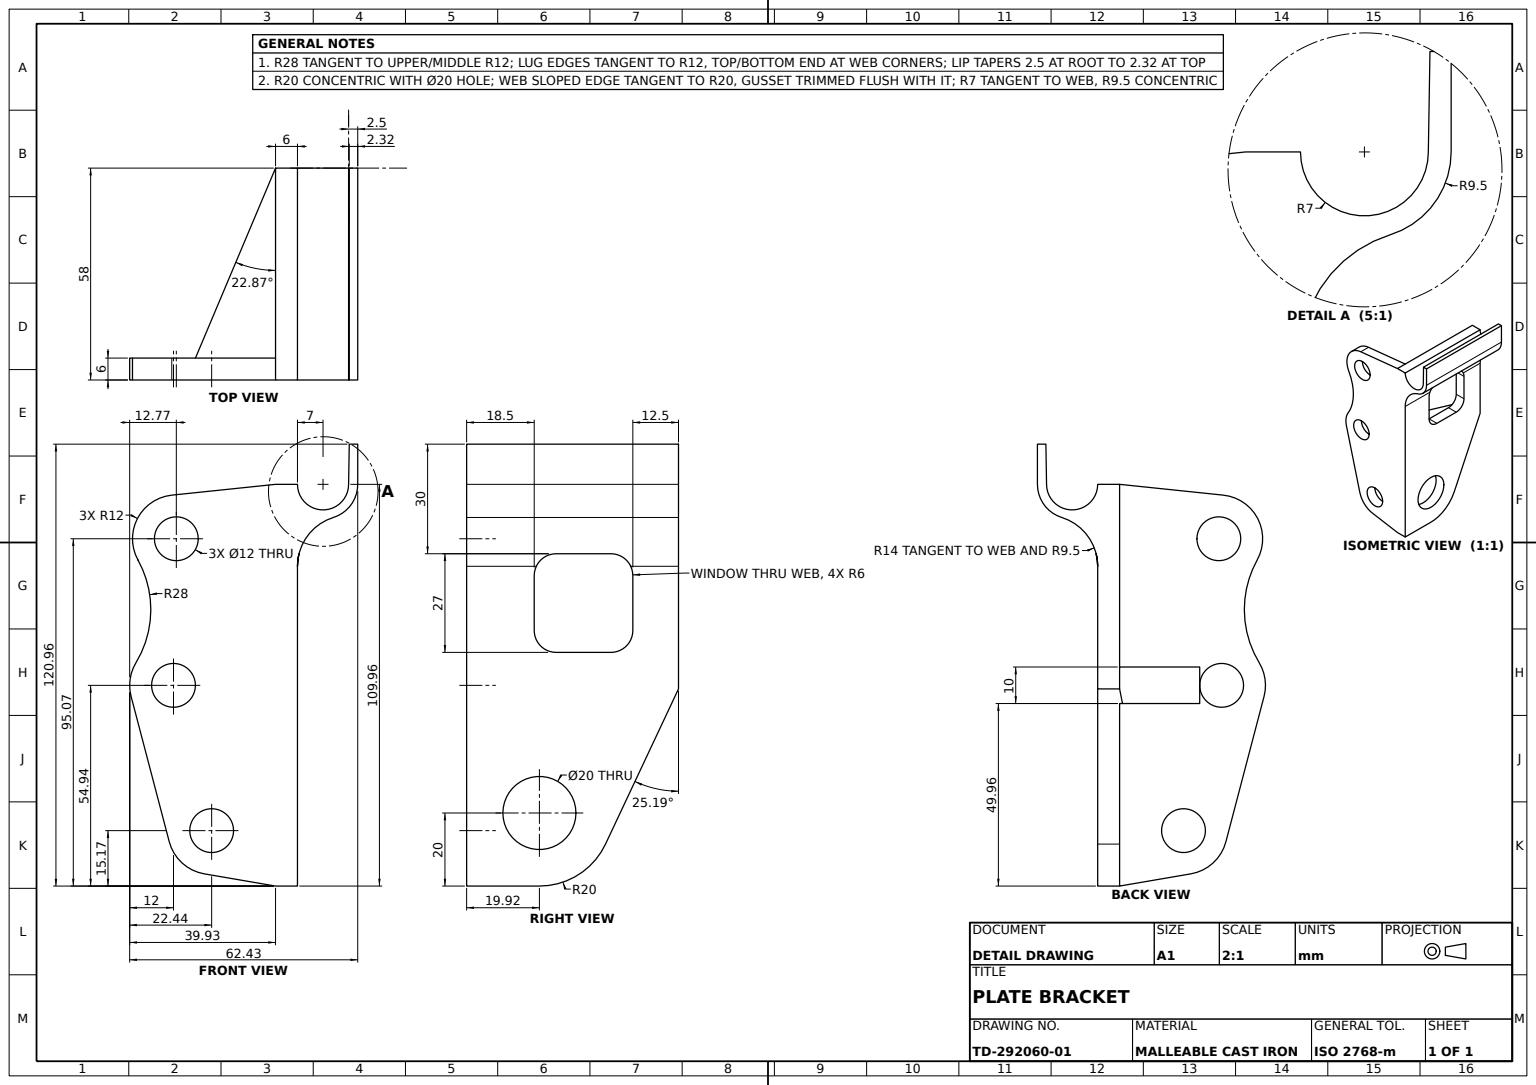
ISO-10303-21;
HEADER;
FILE_DESCRIPTION((''),'2;1');
FILE_NAME('','',(''),(''),'','','');
FILE_SCHEMA(('AUTOMOTIVE_DESIGN'));
ENDSEC;
DATA;
#1=APPLICATION_CONTEXT('');
#2=PRODUCT_CONTEXT('',#1,'mechanical');
#3=PRODUCT('','','',(#2));
#4=PRODUCT_DEFINITION_FORMATION('','',#3);
#5=PRODUCT_DEFINITION_CONTEXT('',#1,'design');
#6=PRODUCT_DEFINITION('','',#4,#5);
#7=PRODUCT_DEFINITION_SHAPE('','',#6);
#8=(LENGTH_UNIT()NAMED_UNIT(*)SI_UNIT(.MILLI.,.METRE.));
#9=(NAMED_UNIT(*)PLANE_ANGLE_UNIT()SI_UNIT($,.RADIAN.));
#10=(NAMED_UNIT(*)SI_UNIT($,.STERADIAN.)SOLID_ANGLE_UNIT());
#11=UNCERTAINTY_MEASURE_WITH_UNIT(LENGTH_MEASURE(1.E-05),#8,'distance_accuracy_value','');
#12=(GEOMETRIC_REPRESENTATION_CONTEXT(3)GLOBAL_UNCERTAINTY_ASSIGNED_CONTEXT((#11))GLOBAL_UNIT_ASSIGNED_CONTEXT((#8,#9,#10))REPRESENTATION_CONTEXT('',''));
#13=CARTESIAN_POINT('',(58.,0.,-14.));
#14=VERTEX_POINT('',#13);
#15=CARTESIAN_POINT('',(58.,0.,0.));
#16=VERTEX_POINT('',#15);
#17=CARTESIAN_POINT('',(58.,0.,-7.));
#18=DIRECTION('',(-1.,0.,0.));
#19=DIRECTION('',(0.,0.,1.));
#20=AXIS2_PLACEMENT_3D('',#17,#18,#19);
#21=CIRCLE('',#20,7.);
#22=EDGE_CURVE('',#14,#16,#21,.T.);
#23=ORIENTED_EDGE('',*,*,#22,.F.);
#24=CARTESIAN_POINT('',(0.,0.,-14.));
#25=VERTEX_POINT('',#24);
#26=VECTOR('',#18,1000.);
#27=LINE('',#13,#26);
#28=EDGE_CURVE('',#14,#25,#27,.T.);
#29=ORIENTED_EDGE('',*,*,#28,.T.);
#30=CARTESIAN_POINT('',(0.,0.,0.));
#31=VERTEX_POINT('',#30);
#32=CARTESIAN_POINT('',(0.,0.,-7.));
#33=AXIS2_PLACEMENT_3D('',#32,#18,#19);
#34=CIRCLE('',#33,7.);
#35=EDGE_CURVE('',#25,#31,#34,.T.);
#36=ORIENTED_EDGE('',*,*,#35,.T.);
#37=LINE('',#15,#26);
#38=EDGE_CURVE('',#16,#31,#37,.T.);
#39=ORIENTED_EDGE('',*,*,#38,.F.);
#40=EDGE_LOOP('',(#23,#29,#36,#39));
#41=FACE_OUTER_BOUND('',#40,.T.);
#42=CYLINDRICAL_SURFACE('',#20,7.);
#43=ADVANCED_FACE('',(#41),#42,.F.);
#44=CARTESIAN_POINT('',(58.,-22.433234,0.));
#45=VERTEX_POINT('',#44);
#46=CARTESIAN_POINT('',(38.923257,-22.433234,0.));
#47=VERTEX_POINT('',#46);
#48=LINE('',#44,#26);
#49=EDGE_CURVE('',#45,#47,#48,.T.);
#50=ORIENTED_EDGE('',*,*,#49,.T.);
#51=CARTESIAN_POINT('',(33.5,-19.,-0.427495));
#52=VERTEX_POINT('',#51);
#53=CARTESIAN_POINT('',(34.070773,-19.,-0.427495));
#54=CARTESIAN_POINT('',(34.627308,-19.07981,-0.406595));
#55=CARTESIAN_POINT('',(35.441627,-19.315816,-0.351255));
#56=CARTESIAN_POINT('',(35.709756,-19.414662,-0.328783));
#57=CARTESIAN_POINT('',(36.222308,-19.645743,-0.279802));
#58=CARTESIAN_POINT('',(36.468987,-19.778515,-0.253156));
#59=CARTESIAN_POINT('',(36.943484,-20.078496,-0.198607));
#60=CARTESIAN_POINT('',(37.172954,-20.247201,-0.170487));
#61=CARTESIAN_POINT('',(37.60295,-20.613033,-0.1176));
#62=CARTESIAN_POINT('',(37.803267,-20.809474,-0.092884));
#63=CARTESIAN_POINT('',(38.361336,-21.438838,-0.028993));
#64=CARTESIAN_POINT('',(38.679064,-21.917284,0.));
#65=B_SPLINE_CURVE_WITH_KNOTS('',3,(#51,#53,#54,#55,#56,#57,#58,#59,#60,#61,#62,#63,#64,#46),.UNSPECIFIED.,.F.,.F.,(4,2,2,2,2,2,4),(0.,0.001687367,0.00253105,0.003374734,0.004218417,0.005062101,0.006749467),.UNSPECIFIED.);
#66=EDGE_CURVE('',#52,#47,#65,.T.);
#67=ORIENTED_EDGE('',*,*,#66,.F.);
#68=CARTESIAN_POINT('',(18.5,-19.,-0.427495));
#69=VERTEX_POINT('',#68);
#70=CARTESIAN_POINT('',(58.,-19.,-0.427495));
#71=DIRECTION('',(1.,0.,0.));
#72=VECTOR('',#71,1000.);
#73=LINE('',#70,#72);
#74=EDGE_CURVE('',#69,#52,#73,.T.);
#75=ORIENTED_EDGE('',*,*,#74,.F.);
#76=CARTESIAN_POINT('',(13.076743,-22.433234,0.));
#77=VERTEX_POINT('',#76);
#78=CARTESIAN_POINT('',(13.320987,-21.917178,0.));
#79=CARTESIAN_POINT('',(13.631064,-21.448593,-0.028194));
#80=CARTESIAN_POINT('',(14.192298,-20.813896,-0.092342));
#81=CARTESIAN_POINT('',(14.396135,-20.613972,-0.117487));
#82=CARTESIAN_POINT('',(14.823977,-20.249653,-0.17011));
#83=CARTESIAN_POINT('',(15.049421,-20.083465,-0.197756));
#84=CARTESIAN_POINT('',(15.523554,-19.782762,-0.252333));
#85=CARTESIAN_POINT('',(15.774331,-19.647385,-0.279463));
#86=CARTESIAN_POINT('',(16.28914,-19.415034,-0.328695));
#87=CARTESIAN_POINT('',(16.55254,-19.317913,-0.350778));
#88=CARTESIAN_POINT('',(17.360605,-19.082516,-0.405933));
#89=CARTESIAN_POINT('',(17.929227,-19.,-0.427495));
#90=B_SPLINE_CURVE_WITH_KNOTS('',3,(#76,#78,#79,#80,#81,#82,#83,#84,#85,#86,#87,#88,#89,#68),.UNSPECIFIED.,.F.,.F.,(4,2,2,2,2,2,4),(0.,0.00168732,0.00253098,0.00337464,0.0042183,0.005061961,0.006749281),.UNSPECIFIED.);
#91=EDGE_CURVE('',#77,#69,#90,.T.);
#92=ORIENTED_EDGE('',*,*,#91,.F.);
#93=CARTESIAN_POINT('',(0.,-22.433234,0.));
#94=VERTEX_POINT('',#93);
#95=EDGE_CURVE('',#77,#94,#48,.T.);
#96=ORIENTED_EDGE('',*,*,#95,.T.);
#97=CARTESIAN_POINT('',(0.,-9.068754,-9.829787));
#98=VERTEX_POINT('',#97);
#99=CARTESIAN_POINT('',(0.,-22.433234,-14.));
#100=DIRECTION('',(0.,0.,-1.));
#101=AXIS2_PLACEMENT_3D('',#99,#71,#100);
#102=CIRCLE('',#101,14.);
#103=EDGE_CURVE('',#98,#94,#102,.T.);
#104=ORIENTED_EDGE('',*,*,#103,.F.);
#105=CARTESIAN_POINT('',(58.,-9.068754,-9.829787));
#106=VERTEX_POINT('',#105);
#107=LINE('',#105,#26);
#108=EDGE_CURVE('',#106,#98,#107,.T.);
#109=ORIENTED_EDGE('',*,*,#108,.F.);
#110=CARTESIAN_POINT('',(58.,-22.433234,-14.));
#111=AXIS2_PLACEMENT_3D('',#110,#71,#100);
#112=CIRCLE('',#111,14.);
#113=EDGE_CURVE('',#106,#45,#112,.T.);
#114=ORIENTED_EDGE('',*,*,#113,.T.);
#115=EDGE_LOOP('',(#50,#67,#75,#92,#96,#104,#109,#114));
#116=FACE_OUTER_BOUND('',#115,.T.);
#117=AXIS2_PLACEMENT_3D('',#110,#18,#19);
#118=CYLINDRICAL_SURFACE('',#117,14.);
#119=ADVANCED_FACE('',(#116),#118,.F.);
#120=CARTESIAN_POINT('',(58.,-97.839179,35.09695));
#121=VERTEX_POINT('',#120);
#122=CARTESIAN_POINT('',(58.,-106.618686,25.517753));
#123=VERTEX_POINT('',#122);
#124=CARTESIAN_POINT('',(58.,-94.791164,23.490503));
#125=AXIS2_PLACEMENT_3D('',#124,#71,#100);
#126=CIRCLE('',#125,12.);
#127=EDGE_CURVE('',#121,#123,#126,.T.);
#128=ORIENTED_EDGE('',*,*,#127,.F.);
#129=CARTESIAN_POINT('',(52.,-97.839179,35.09695));
#130=VERTEX_POINT('',#129);
#131=LINE('',#129,#72);
#132=EDGE_CURVE('',#130,#121,#131,.T.);
#133=ORIENTED_EDGE('',*,*,#132,.F.);
#134=CARTESIAN_POINT('',(52.,-106.618686,25.517753));
#135=VERTEX_POINT('',#134);
#136=CARTESIAN_POINT('',(52.,-94.791164,23.490503));
#137=AXIS2_PLACEMENT_3D('',#136,#71,#100);
#138=CIRCLE('',#137,12.);
#139=EDGE_CURVE('',#130,#135,#138,.T.);
#140=ORIENTED_EDGE('',*,*,#139,.T.);
#141=LINE('',#134,#72);
#142=EDGE_CURVE('',#135,#123,#141,.T.);
#143=ORIENTED_EDGE('',*,*,#142,.T.);
#144=EDGE_LOOP('',(#128,#133,#140,#143));
#145=FACE_OUTER_BOUND('',#144,.T.);
#146=CYLINDRICAL_SURFACE('',#137,12.);
#147=ADVANCED_FACE('',(#145),#146,.T.);
#148=CARTESIAN_POINT('',(58.,0.,-16.5));
#149=VERTEX_POINT('',#148);
#150=CIRCLE('',#20,9.5);
#151=EDGE_CURVE('',#149,#106,#150,.T.);
#152=ORIENTED_EDGE('',*,*,#151,.T.);
#153=ORIENTED_EDGE('',*,*,#108,.T.);
#154=CARTESIAN_POINT('',(0.,0.,-16.5));
#155=VERTEX_POINT('',#154);
#156=CIRCLE('',#33,9.5);
#157=EDGE_CURVE('',#155,#98,#156,.T.);
#158=ORIENTED_EDGE('',*,*,#157,.F.);
#159=LINE('',#148,#26);
#160=EDGE_CURVE('',#149,#155,#159,.T.);
#161=ORIENTED_EDGE('',*,*,#160,.F.);
#162=EDGE_LOOP('',(#152,#153,#158,#161));
#163=FACE_OUTER_BOUND('',#162,.T.);
#164=CYLINDRICAL_SURFACE('',#20,9.5);
#165=ADVANCED_FACE('',(#163),#164,.T.);
#166=CARTESIAN_POINT('',(48.076435,-89.96405,0.));
#167=VERTEX_POINT('',#166);
#168=CARTESIAN_POINT('',(28.076435,-89.96405,0.));
#169=VERTEX_POINT('',#168);
#170=CARTESIAN_POINT('',(38.076435,-89.96405,0.));
#171=AXIS2_PLACEMENT_3D('',#170,#19,#71);
#172=CIRCLE('',#171,10.);
#173=EDGE_CURVE('',#167,#169,#172,.T.);
#174=ORIENTED_EDGE('',*,*,#173,.F.);
#175=CARTESIAN_POINT('',(48.076435,-89.96405,6.));
#176=VERTEX_POINT('',#175);
#177=VECTOR('',#19,1000.);
#178=LINE('',#166,#177);
#179=EDGE_CURVE('',#167,#176,#178,.T.);
#180=ORIENTED_EDGE('',*,*,#179,.T.);
#181=CARTESIAN_POINT('',(28.076435,-89.96405,6.));
#182=VERTEX_POINT('',#181);
#183=CARTESIAN_POINT('',(38.076435,-89.96405,6.));
#184=AXIS2_PLACEMENT_3D('',#183,#19,#71);
#185=CIRCLE('',#184,10.);
#186=EDGE_CURVE('',#176,#182,#185,.T.);
#187=ORIENTED_EDGE('',*,*,#186,.T.);
#188=LINE('',#168,#177);
#189=EDGE_CURVE('',#169,#182,#188,.T.);
#190=ORIENTED_EDGE('',*,*,#189,.F.);
#191=EDGE_LOOP('',(#174,#180,#187,#190));
#192=FACE_OUTER_BOUND('',#191,.T.);
#193=CYLINDRICAL_SURFACE('',#171,10.);
#194=ADVANCED_FACE('',(#192),#193,.F.);
#195=CARTESIAN_POINT('',(12.5,-40.,0.));
#196=VERTEX_POINT('',#195);
#197=CARTESIAN_POINT('',(12.5,-40.,6.));
#198=VERTEX_POINT('',#197);
#199=LINE('',#195,#177);
#200=EDGE_CURVE('',#196,#198,#199,.T.);
#201=ORIENTED_EDGE('',*,*,#200,.T.);
#202=CARTESIAN_POINT('',(18.5,-46.,6.));
#203=VERTEX_POINT('',#202);
#204=CARTESIAN_POINT('',(18.5,-40.,6.));
#205=AXIS2_PLACEMENT_3D('',#204,#19,#18);
#206=CIRCLE('',#205,6.);
#207=EDGE_CURVE('',#198,#203,#206,.T.);
#208=ORIENTED_EDGE('',*,*,#207,.T.);
#209=CARTESIAN_POINT('',(18.5,-46.,0.));
#210=VERTEX_POINT('',#209);
#211=LINE('',#209,#177);
#212=EDGE_CURVE('',#210,#203,#211,.T.);
#213=ORIENTED_EDGE('',*,*,#212,.F.);
#214=CARTESIAN_POINT('',(18.5,-40.,0.));
#215=AXIS2_PLACEMENT_3D('',#214,#19,#18);
#216=CIRCLE('',#215,6.);
#217=EDGE_CURVE('',#196,#210,#216,.T.);
#218=ORIENTED_EDGE('',*,*,#217,.F.);
#219=EDGE_LOOP('',(#201,#208,#213,#218));
#220=FACE_OUTER_BOUND('',#219,.T.);
#221=AXIS2_PLACEMENT_3D('',#214,#19,#71);
#222=CYLINDRICAL_SURFACE('',#221,6.);
#223=ADVANCED_FACE('',(#220),#222,.F.);
#224=CARTESIAN_POINT('',(58.,-55.021696,27.934519));
#225=VERTEX_POINT('',#224);
#226=CARTESIAN_POINT('',(52.,-55.021696,27.934519));
#227=VERTEX_POINT('',#226);
#228=LINE('',#224,#26);
#229=EDGE_CURVE('',#225,#227,#228,.T.);
#230=ORIENTED_EDGE('',*,*,#229,.F.);
#231=CARTESIAN_POINT('',(58.,-55.021696,39.934519));
#232=VERTEX_POINT('',#231);
#233=CARTESIAN_POINT('',(58.,-55.021696,33.934519));
#234=AXIS2_PLACEMENT_3D('',#233,#18,#19);
#235=CIRCLE('',#234,6.);
#236=EDGE_CURVE('',#232,#225,#235,.T.);
#237=ORIENTED_EDGE('',*,*,#236,.F.);
#238=CARTESIAN_POINT('',(52.,-55.021696,39.934519));
#239=VERTEX_POINT('',#238);
#240=LINE('',#231,#26);
#241=EDGE_CURVE('',#232,#239,#240,.T.);
#242=ORIENTED_EDGE('',*,*,#241,.T.);
#243=CARTESIAN_POINT('',(52.,-55.021696,33.934519));
#244=AXIS2_PLACEMENT_3D('',#243,#18,#19);
#245=CIRCLE('',#244,6.);
#246=EDGE_CURVE('',#239,#227,#245,.T.);
#247=ORIENTED_EDGE('',*,*,#246,.T.);
#248=EDGE_LOOP('',(#230,#237,#242,#247));
#249=FACE_OUTER_BOUND('',#248,.T.);
#250=CYLINDRICAL_SURFACE('',#234,6.);
#251=ADVANCED_FACE('',(#249),#250,.F.);
#252=ORIENTED_EDGE('',*,*,#173,.T.);
#253=EDGE_CURVE('',#169,#167,#172,.T.);
#254=ORIENTED_EDGE('',*,*,#253,.T.);
#255=EDGE_LOOP('',(#252,#254));
#256=FACE_BOUND('',#255,.T.);
#257=CARTESIAN_POINT('',(19.978333,-98.47632,0.));
#258=VERTEX_POINT('',#257);
#259=CARTESIAN_POINT('',(38.076435,-109.96405,0.));
#260=VERTEX_POINT('',#259);
#261=CIRCLE('',#171,20.);
#262=EDGE_CURVE('',#258,#260,#261,.T.);
#263=ORIENTED_EDGE('',*,*,#262,.F.);
#264=CARTESIAN_POINT('',(0.,-56.,0.));
#265=VERTEX_POINT('',#264);
#266=CARTESIAN_POINT('',(-21.567829,-10.144223,0.));
#267=DIRECTION('',(0.425613496,-0.904905052,0.));
#268=VECTOR('',#267,1000.);
#269=LINE('',#266,#268);
#270=EDGE_CURVE('',#265,#258,#269,.T.);
#271=ORIENTED_EDGE('',*,*,#270,.F.);
#272=DIRECTION('',(0.,-1.,0.));
#273=VECTOR('',#272,1000.);
#274=LINE('',#30,#273);
#275=EDGE_CURVE('',#94,#265,#274,.T.);
#276=ORIENTED_EDGE('',*,*,#275,.F.);
#277=ORIENTED_EDGE('',*,*,#95,.F.);
#278=CARTESIAN_POINT('',(12.5,-25.,0.));
#279=VERTEX_POINT('',#278);
#280=CARTESIAN_POINT('',(18.5,-25.,0.));
#281=AXIS2_PLACEMENT_3D('',#280,#19,#18);
#282=CIRCLE('',#281,6.);
#283=EDGE_CURVE('',#77,#279,#282,.T.);
#284=ORIENTED_EDGE('',*,*,#283,.T.);
#285=LINE('',#195,#273);
#286=EDGE_CURVE('',#279,#196,#285,.T.);
#287=ORIENTED_EDGE('',*,*,#286,.T.);
#288=ORIENTED_EDGE('',*,*,#217,.T.);
#289=CARTESIAN_POINT('',(33.5,-46.,0.));
#290=VERTEX_POINT('',#289);
#291=LINE('',#209,#72);
#292=EDGE_CURVE('',#210,#290,#291,.T.);
#293=ORIENTED_EDGE('',*,*,#292,.T.);
#294=CARTESIAN_POINT('',(39.5,-40.,0.));
#295=VERTEX_POINT('',#294);
#296=CARTESIAN_POINT('',(33.5,-40.,0.));
#297=AXIS2_PLACEMENT_3D('',#296,#19,#71);
#298=CIRCLE('',#297,6.);
#299=EDGE_CURVE('',#290,#295,#298,.T.);
#300=ORIENTED_EDGE('',*,*,#299,.T.);
#301=CARTESIAN_POINT('',(39.5,-25.,0.));
#302=VERTEX_POINT('',#301);
#303=DIRECTION('',(0.,1.,0.));
#304=VECTOR('',#303,1000.);
#305=LINE('',#301,#304);
#306=EDGE_CURVE('',#295,#302,#305,.T.);
#307=ORIENTED_EDGE('',*,*,#306,.T.);
#308=CARTESIAN_POINT('',(33.5,-25.,0.));
#309=AXIS2_PLACEMENT_3D('',#308,#19,#71);
#310=CIRCLE('',#309,6.);
#311=EDGE_CURVE('',#302,#47,#310,.T.);
#312=ORIENTED_EDGE('',*,*,#311,.T.);
#313=ORIENTED_EDGE('',*,*,#49,.F.);
#314=CARTESIAN_POINT('',(58.,-109.96405,0.));
#315=VERTEX_POINT('',#314);
#316=LINE('',#15,#304);
#317=EDGE_CURVE('',#315,#45,#316,.T.);
#318=ORIENTED_EDGE('',*,*,#317,.F.);
#319=CARTESIAN_POINT('',(0.,-109.96405,0.));
#320=LINE('',#319,#26);
#321=EDGE_CURVE('',#315,#260,#320,.T.);
#322=ORIENTED_EDGE('',*,*,#321,.T.);
#323=EDGE_LOOP('',(#263,#271,#276,#277,#284,#287,#288,#293,#300,#307,#312,#313,#318,#322));
#324=FACE_OUTER_BOUND('',#323,.T.);
#325=AXIS2_PLACEMENT_3D('',#30,#19,#71);
#326=PLANE('',#325);
#327=ADVANCED_FACE('',(#256,#324),#326,.F.);
#328=CARTESIAN_POINT('',(18.5,-19.,6.));
#329=VERTEX_POINT('',#328);
#330=CARTESIAN_POINT('',(18.5,-19.,0.));
#331=LINE('',#330,#177);
#332=EDGE_CURVE('',#69,#329,#331,.T.);
#333=ORIENTED_EDGE('',*,*,#332,.T.);
#334=CARTESIAN_POINT('',(12.5,-25.,6.));
#335=VERTEX_POINT('',#334);
#336=CARTESIAN_POINT('',(18.5,-25.,6.));
#337=AXIS2_PLACEMENT_3D('',#336,#19,#18);
#338=CIRCLE('',#337,6.);
#339=EDGE_CURVE('',#329,#335,#338,.T.);
#340=ORIENTED_EDGE('',*,*,#339,.T.);
#341=LINE('',#278,#177);
#342=EDGE_CURVE('',#279,#335,#341,.T.);
#343=ORIENTED_EDGE('',*,*,#342,.F.);
#344=ORIENTED_EDGE('',*,*,#283,.F.);
#345=ORIENTED_EDGE('',*,*,#91,.T.);
#346=EDGE_LOOP('',(#333,#340,#343,#344,#345));
#347=FACE_OUTER_BOUND('',#346,.T.);
#348=AXIS2_PLACEMENT_3D('',#280,#19,#71);
#349=CYLINDRICAL_SURFACE('',#348,6.);
#350=ADVANCED_FACE('',(#347),#349,.F.);
#351=CARTESIAN_POINT('',(52.,-94.791164,17.490503));
#352=VERTEX_POINT('',#351);
#353=CARTESIAN_POINT('',(52.,-94.791164,29.490503));
#354=VERTEX_POINT('',#353);
#355=AXIS2_PLACEMENT_3D('',#136,#18,#19);
#356=CIRCLE('',#355,6.);
#357=EDGE_CURVE('',#352,#354,#356,.T.);
#358=ORIENTED_EDGE('',*,*,#357,.T.);
#359=CARTESIAN_POINT('',(58.,-94.791164,29.490503));
#360=VERTEX_POINT('',#359);
#361=LINE('',#359,#26);
#362=EDGE_CURVE('',#360,#354,#361,.T.);
#363=ORIENTED_EDGE('',*,*,#362,.F.);
#364=CARTESIAN_POINT('',(58.,-94.791164,17.490503));
#365=VERTEX_POINT('',#364);
#366=AXIS2_PLACEMENT_3D('',#124,#18,#19);
#367=CIRCLE('',#366,6.);
#368=EDGE_CURVE('',#365,#360,#367,.T.);
#369=ORIENTED_EDGE('',*,*,#368,.F.);
#370=LINE('',#364,#26);
#371=EDGE_CURVE('',#365,#352,#370,.T.);
#372=ORIENTED_EDGE('',*,*,#371,.T.);
#373=EDGE_LOOP('',(#358,#363,#369,#372));
#374=FACE_OUTER_BOUND('',#373,.T.);
#375=CYLINDRICAL_SURFACE('',#366,6.);
#376=ADVANCED_FACE('',(#374),#375,.F.);
#377=ORIENTED_EDGE('',*,*,#246,.F.);
#378=EDGE_CURVE('',#227,#239,#245,.T.);
#379=ORIENTED_EDGE('',*,*,#378,.F.);
#380=EDGE_LOOP('',(#377,#379));
#381=FACE_BOUND('',#380,.T.);
#382=CARTESIAN_POINT('',(52.,-20.715004,43.659208));
#383=VERTEX_POINT('',#382);
#384=CARTESIAN_POINT('',(52.,-34.294929,40.145645));
#385=VERTEX_POINT('',#384);
#386=CARTESIAN_POINT('',(52.,-34.294929,68.145645));
#387=AXIS2_PLACEMENT_3D('',#386,#18,#19);
#388=CIRCLE('',#387,28.);
#389=EDGE_CURVE('',#383,#385,#388,.T.);
#390=ORIENTED_EDGE('',*,*,#389,.F.);
#391=CARTESIAN_POINT('',(52.,-2.959633,34.408467));
#392=VERTEX_POINT('',#391);
#393=CARTESIAN_POINT('',(52.,-14.895036,33.16502));
#394=AXIS2_PLACEMENT_3D('',#393,#71,#100);
#395=CIRCLE('',#394,12.);
#396=EDGE_CURVE('',#392,#383,#395,.T.);
#397=ORIENTED_EDGE('',*,*,#396,.F.);
#398=CARTESIAN_POINT('',(52.,0.,6.));
#399=VERTEX_POINT('',#398);
#400=DIRECTION('',(0.,-0.103620542,0.994616903));
#401=VECTOR('',#400,1000.);
#402=LINE('',#398,#401);
#403=EDGE_CURVE('',#399,#392,#402,.T.);
#404=ORIENTED_EDGE('',*,*,#403,.F.);
#405=CARTESIAN_POINT('',(52.,-50.,6.));
#406=VERTEX_POINT('',#405);
#407=LINE('',#405,#304);
#408=EDGE_CURVE('',#406,#399,#407,.T.);
#409=ORIENTED_EDGE('',*,*,#408,.F.);
#410=CARTESIAN_POINT('',(52.,-50.,27.93));
#411=VERTEX_POINT('',#410);
#412=VECTOR('',#100,1000.);
#413=LINE('',#405,#412);
#414=EDGE_CURVE('',#411,#406,#413,.T.);
#415=ORIENTED_EDGE('',*,*,#414,.F.);
#416=CARTESIAN_POINT('',(52.,-60.,27.93));
#417=VERTEX_POINT('',#416);
#418=LINE('',#416,#304);
#419=EDGE_CURVE('',#417,#411,#418,.T.);
#420=ORIENTED_EDGE('',*,*,#419,.F.);
#421=CARTESIAN_POINT('',(52.,-60.,6.));
#422=VERTEX_POINT('',#421);
#423=LINE('',#421,#412);
#424=EDGE_CURVE('',#417,#422,#423,.T.);
#425=ORIENTED_EDGE('',*,*,#424,.T.);
#426=CARTESIAN_POINT('',(52.,-109.96405,6.));
#427=VERTEX_POINT('',#426);
#428=LINE('',#398,#304);
#429=EDGE_CURVE('',#427,#422,#428,.T.);
#430=ORIENTED_EDGE('',*,*,#429,.F.);
#431=DIRECTION('',(0.,-0.168937496,-0.985626766));
#432=VECTOR('',#431,1000.);
#433=LINE('',#426,#432);
#434=EDGE_CURVE('',#135,#427,#433,.T.);
#435=ORIENTED_EDGE('',*,*,#434,.F.);
#436=ORIENTED_EDGE('',*,*,#139,.F.);
#437=CARTESIAN_POINT('',(52.,-58.069711,45.540966));
#438=VERTEX_POINT('',#437);
#439=DIRECTION('',(0.,-0.967203903,-0.254001202));
#440=VECTOR('',#439,1000.);
#441=LINE('',#437,#440);
#442=EDGE_CURVE('',#438,#130,#441,.T.);
#443=ORIENTED_EDGE('',*,*,#442,.F.);
#444=CARTESIAN_POINT('',(52.,-48.803666,44.197857));
#445=VERTEX_POINT('',#444);
#446=AXIS2_PLACEMENT_3D('',#243,#71,#100);
#447=CIRCLE('',#446,12.);
#448=EDGE_CURVE('',#445,#438,#447,.T.);
#449=ORIENTED_EDGE('',*,*,#448,.F.);
#450=EDGE_CURVE('',#385,#445,#388,.T.);
#451=ORIENTED_EDGE('',*,*,#450,.F.);
#452=EDGE_LOOP('',(#390,#397,#404,#409,#415,#420,#425,#430,#435,#436,#443,#449,#451));
#453=FACE_OUTER_BOUND('',#452,.T.);
#454=CARTESIAN_POINT('',(52.,-14.895036,39.16502));
#455=VERTEX_POINT('',#454);
#456=CARTESIAN_POINT('',(52.,-14.895036,27.16502));
#457=VERTEX_POINT('',#456);
#458=AXIS2_PLACEMENT_3D('',#393,#18,#19);
#459=CIRCLE('',#458,6.);
#460=EDGE_CURVE('',#455,#457,#459,.T.);
#461=ORIENTED_EDGE('',*,*,#460,.F.);
#462=EDGE_CURVE('',#457,#455,#459,.T.);
#463=ORIENTED_EDGE('',*,*,#462,.F.);
#464=EDGE_LOOP('',(#461,#463));
#465=FACE_BOUND('',#464,.T.);
#466=ORIENTED_EDGE('',*,*,#357,.F.);
#467=EDGE_CURVE('',#354,#352,#356,.T.);
#468=ORIENTED_EDGE('',*,*,#467,.F.);
#469=EDGE_LOOP('',(#466,#468));
#470=FACE_BOUND('',#469,.T.);
#471=PLANE('',#394);
#472=ADVANCED_FACE('',(#381,#453,#465,#470),#471,.F.);
#473=CARTESIAN_POINT('',(0.,0.,6.));
#474=VERTEX_POINT('',#473);
#475=LINE('',#473,#26);
#476=EDGE_CURVE('',#399,#474,#475,.T.);
#477=ORIENTED_EDGE('',*,*,#476,.F.);
#478=CARTESIAN_POINT('',(58.,0.,6.));
#479=VERTEX_POINT('',#478);
#480=EDGE_CURVE('',#479,#399,#475,.T.);
#481=ORIENTED_EDGE('',*,*,#480,.F.);
#482=LINE('',#478,#412);
#483=EDGE_CURVE('',#479,#16,#482,.T.);
#484=ORIENTED_EDGE('',*,*,#483,.T.);
#485=ORIENTED_EDGE('',*,*,#38,.T.);
#486=LINE('',#473,#412);
#487=EDGE_CURVE('',#474,#31,#486,.T.);
#488=ORIENTED_EDGE('',*,*,#487,.F.);
#489=EDGE_LOOP('',(#477,#481,#484,#485,#488));
#490=FACE_OUTER_BOUND('',#489,.T.);
#491=AXIS2_PLACEMENT_3D('',#473,#272,#100);
#492=PLANE('',#491);
#493=ADVANCED_FACE('',(#490),#492,.F.);
#494=CARTESIAN_POINT('',(33.5,-46.,6.));
#495=VERTEX_POINT('',#494);
#496=CARTESIAN_POINT('',(39.5,-40.,6.));
#497=VERTEX_POINT('',#496);
#498=CARTESIAN_POINT('',(33.5,-40.,6.));
#499=AXIS2_PLACEMENT_3D('',#498,#19,#71);
#500=CIRCLE('',#499,6.);
#501=EDGE_CURVE('',#495,#497,#500,.T.);
#502=ORIENTED_EDGE('',*,*,#501,.F.);
#503=LINE('',#202,#72);
#504=EDGE_CURVE('',#203,#495,#503,.T.);
#505=ORIENTED_EDGE('',*,*,#504,.F.);
#506=ORIENTED_EDGE('',*,*,#207,.F.);
#507=LINE('',#197,#273);
#508=EDGE_CURVE('',#335,#198,#507,.T.);
#509=ORIENTED_EDGE('',*,*,#508,.F.);
#510=ORIENTED_EDGE('',*,*,#339,.F.);
#511=CARTESIAN_POINT('',(33.5,-19.,6.));
#512=VERTEX_POINT('',#511);
#513=LINE('',#328,#26);
#514=EDGE_CURVE('',#512,#329,#513,.T.);
#515=ORIENTED_EDGE('',*,*,#514,.F.);
#516=CARTESIAN_POINT('',(39.5,-25.,6.));
#517=VERTEX_POINT('',#516);
#518=CARTESIAN_POINT('',(33.5,-25.,6.));
#519=AXIS2_PLACEMENT_3D('',#518,#19,#71);
#520=CIRCLE('',#519,6.);
#521=EDGE_CURVE('',#517,#512,#520,.T.);
#522=ORIENTED_EDGE('',*,*,#521,.F.);
#523=LINE('',#516,#304);
#524=EDGE_CURVE('',#497,#517,#523,.T.);
#525=ORIENTED_EDGE('',*,*,#524,.F.);
#526=EDGE_LOOP('',(#502,#505,#506,#509,#510,#515,#522,#525));
#527=FACE_BOUND('',#526,.T.);
#528=ORIENTED_EDGE('',*,*,#476,.T.);
#529=CARTESIAN_POINT('',(0.,-50.,6.));
#530=VERTEX_POINT('',#529);
#531=LINE('',#473,#273);
#532=EDGE_CURVE('',#474,#530,#531,.T.);
#533=ORIENTED_EDGE('',*,*,#532,.T.);
#534=LINE('',#529,#26);
#535=EDGE_CURVE('',#406,#530,#534,.T.);
#536=ORIENTED_EDGE('',*,*,#535,.F.);
#537=ORIENTED_EDGE('',*,*,#408,.T.);
#538=EDGE_LOOP('',(#528,#533,#536,#537));
#539=FACE_OUTER_BOUND('',#538,.T.);
#540=AXIS2_PLACEMENT_3D('',#529,#100,#18);
#541=PLANE('',#540);
#542=ADVANCED_FACE('',(#527,#539),#541,.F.);
#543=CARTESIAN_POINT('',(38.076435,-109.96405,6.));
#544=VERTEX_POINT('',#543);
#545=LINE('',#259,#177);
#546=EDGE_CURVE('',#260,#544,#545,.T.);
#547=ORIENTED_EDGE('',*,*,#546,.F.);
#548=ORIENTED_EDGE('',*,*,#321,.F.);
#549=CARTESIAN_POINT('',(58.,-109.96405,6.));
#550=VERTEX_POINT('',#549);
#551=LINE('',#314,#177);
#552=EDGE_CURVE('',#315,#550,#551,.T.);
#553=ORIENTED_EDGE('',*,*,#552,.T.);
#554=CARTESIAN_POINT('',(0.,-109.96405,6.));
#555=LINE('',#554,#26);
#556=EDGE_CURVE('',#550,#427,#555,.T.);
#557=ORIENTED_EDGE('',*,*,#556,.T.);
#558=EDGE_CURVE('',#427,#544,#555,.T.);
#559=ORIENTED_EDGE('',*,*,#558,.T.);
#560=EDGE_LOOP('',(#547,#548,#553,#557,#559));
#561=FACE_OUTER_BOUND('',#560,.T.);
#562=AXIS2_PLACEMENT_3D('',#319,#303,#18);
#563=PLANE('',#562);
#564=ADVANCED_FACE('',(#561),#563,.F.);
#565=ORIENTED_EDGE('',*,*,#189,.T.);
#566=EDGE_CURVE('',#182,#176,#185,.T.);
#567=ORIENTED_EDGE('',*,*,#566,.T.);
#568=ORIENTED_EDGE('',*,*,#179,.F.);
#569=ORIENTED_EDGE('',*,*,#253,.F.);
#570=EDGE_LOOP('',(#565,#567,#568,#569));
#571=FACE_OUTER_BOUND('',#570,.T.);
#572=ADVANCED_FACE('',(#571),#193,.F.);
#573=CARTESIAN_POINT('',(58.,-2.959633,34.408467));
#574=VERTEX_POINT('',#573);
#575=CARTESIAN_POINT('',(58.,-20.715004,43.659208));
#576=VERTEX_POINT('',#575);
#577=CARTESIAN_POINT('',(58.,-14.895036,33.16502));
#578=AXIS2_PLACEMENT_3D('',#577,#71,#100);
#579=CIRCLE('',#578,12.);
#580=EDGE_CURVE('',#574,#576,#579,.T.);
#581=ORIENTED_EDGE('',*,*,#580,.F.);
#582=LINE('',#391,#72);
#583=EDGE_CURVE('',#392,#574,#582,.T.);
#584=ORIENTED_EDGE('',*,*,#583,.F.);
#585=ORIENTED_EDGE('',*,*,#396,.T.);
#586=LINE('',#382,#72);
#587=EDGE_CURVE('',#383,#576,#586,.T.);
#588=ORIENTED_EDGE('',*,*,#587,.T.);
#589=EDGE_LOOP('',(#581,#584,#585,#588));
#590=FACE_OUTER_BOUND('',#589,.T.);
#591=CYLINDRICAL_SURFACE('',#394,12.);
#592=ADVANCED_FACE('',(#590),#591,.T.);
#593=ORIENTED_EDGE('',*,*,#480,.T.);
#594=ORIENTED_EDGE('',*,*,#403,.T.);
#595=ORIENTED_EDGE('',*,*,#583,.T.);
#596=LINE('',#478,#401);
#597=EDGE_CURVE('',#479,#574,#596,.T.);
#598=ORIENTED_EDGE('',*,*,#597,.F.);
#599=EDGE_LOOP('',(#593,#594,#595,#598));
#600=FACE_OUTER_BOUND('',#599,.T.);
#601=DIRECTION('',(0.,0.994616903,0.103620542));
#602=AXIS2_PLACEMENT_3D('',#398,#601,#400);
#603=PLANE('',#602);
#604=ADVANCED_FACE('',(#600),#603,.T.);
#605=CARTESIAN_POINT('',(58.,-34.294929,40.145645));
#606=VERTEX_POINT('',#605);
#607=CARTESIAN_POINT('',(58.,-34.294929,68.145645));
#608=AXIS2_PLACEMENT_3D('',#607,#18,#19);
#609=CIRCLE('',#608,28.);
#610=EDGE_CURVE('',#576,#606,#609,.T.);
#611=ORIENTED_EDGE('',*,*,#610,.F.);
#612=ORIENTED_EDGE('',*,*,#587,.F.);
#613=ORIENTED_EDGE('',*,*,#389,.T.);
#614=LINE('',#384,#72);
#615=EDGE_CURVE('',#385,#606,#614,.T.);
#616=ORIENTED_EDGE('',*,*,#615,.T.);
#617=EDGE_LOOP('',(#611,#612,#613,#616));
#618=FACE_OUTER_BOUND('',#617,.T.);
#619=AXIS2_PLACEMENT_3D('',#386,#71,#100);
#620=CYLINDRICAL_SURFACE('',#619,28.);
#621=ADVANCED_FACE('',(#618),#620,.F.);
#622=ORIENTED_EDGE('',*,*,#508,.T.);
#623=ORIENTED_EDGE('',*,*,#200,.F.);
#624=ORIENTED_EDGE('',*,*,#286,.F.);
#625=ORIENTED_EDGE('',*,*,#342,.T.);
#626=EDGE_LOOP('',(#622,#623,#624,#625));
#627=FACE_OUTER_BOUND('',#626,.T.);
#628=AXIS2_PLACEMENT_3D('',#195,#18,#19);
#629=PLANE('',#628);
#630=ADVANCED_FACE('',(#627),#629,.F.);
#631=ORIENTED_EDGE('',*,*,#514,.T.);
#632=ORIENTED_EDGE('',*,*,#332,.F.);
#633=ORIENTED_EDGE('',*,*,#74,.T.);
#634=CARTESIAN_POINT('',(33.5,-19.,0.));
#635=LINE('',#634,#177);
#636=EDGE_CURVE('',#52,#512,#635,.T.);
#637=ORIENTED_EDGE('',*,*,#636,.T.);
#638=EDGE_LOOP('',(#631,#632,#633,#637));
#639=FACE_OUTER_BOUND('',#638,.T.);
#640=AXIS2_PLACEMENT_3D('',#330,#303,#18);
#641=PLANE('',#640);
#642=ADVANCED_FACE('',(#639),#641,.F.);
#643=ORIENTED_EDGE('',*,*,#22,.T.);
#644=ORIENTED_EDGE('',*,*,#483,.F.);
#645=ORIENTED_EDGE('',*,*,#597,.T.);
#646=ORIENTED_EDGE('',*,*,#580,.T.);
#647=ORIENTED_EDGE('',*,*,#610,.T.);
#648=CARTESIAN_POINT('',(58.,-48.803666,44.197857));
#649=VERTEX_POINT('',#648);
#650=EDGE_CURVE('',#606,#649,#609,.T.);
#651=ORIENTED_EDGE('',*,*,#650,.T.);
#652=CARTESIAN_POINT('',(58.,-58.069711,45.540966));
#653=VERTEX_POINT('',#652);
#654=AXIS2_PLACEMENT_3D('',#233,#71,#100);
#655=CIRCLE('',#654,12.);
#656=EDGE_CURVE('',#649,#653,#655,.T.);
#657=ORIENTED_EDGE('',*,*,#656,.T.);
#658=LINE('',#652,#440);
#659=EDGE_CURVE('',#653,#121,#658,.T.);
#660=ORIENTED_EDGE('',*,*,#659,.T.);
#661=ORIENTED_EDGE('',*,*,#127,.T.);
#662=LINE('',#549,#432);
#663=EDGE_CURVE('',#123,#550,#662,.T.);
#664=ORIENTED_EDGE('',*,*,#663,.T.);
#665=ORIENTED_EDGE('',*,*,#552,.F.);
#666=ORIENTED_EDGE('',*,*,#317,.T.);
#667=ORIENTED_EDGE('',*,*,#113,.F.);
#668=ORIENTED_EDGE('',*,*,#151,.F.);
#669=CARTESIAN_POINT('',(58.,11.,-16.5));
#670=VERTEX_POINT('',#669);
#671=LINE('',#148,#273);
#672=EDGE_CURVE('',#670,#149,#671,.T.);
#673=ORIENTED_EDGE('',*,*,#672,.F.);
#674=CARTESIAN_POINT('',(58.,11.,-14.17924));
#675=VERTEX_POINT('',#674);
#676=LINE('',#669,#412);
#677=EDGE_CURVE('',#675,#670,#676,.T.);
#678=ORIENTED_EDGE('',*,*,#677,.F.);
#679=DIRECTION('',(0.,0.99986727,-0.016292425));
#680=VECTOR('',#679,1000.);
#681=LINE('',#674,#680);
#682=EDGE_CURVE('',#14,#675,#681,.T.);
#683=ORIENTED_EDGE('',*,*,#682,.F.);
#684=EDGE_LOOP('',(#643,#644,#645,#646,#647,#651,#657,#660,#661,#664,#665,#666,#667,#668,#673,#678,#683));
#685=FACE_OUTER_BOUND('',#684,.T.);
#686=EDGE_CURVE('',#360,#365,#367,.T.);
#687=ORIENTED_EDGE('',*,*,#686,.T.);
#688=ORIENTED_EDGE('',*,*,#368,.T.);
#689=EDGE_LOOP('',(#687,#688));
#690=FACE_BOUND('',#689,.T.);
#691=EDGE_CURVE('',#225,#232,#235,.T.);
#692=ORIENTED_EDGE('',*,*,#691,.T.);
#693=ORIENTED_EDGE('',*,*,#236,.T.);
#694=EDGE_LOOP('',(#692,#693));
#695=FACE_BOUND('',#694,.T.);
#696=CARTESIAN_POINT('',(58.,-14.895036,27.16502));
#697=VERTEX_POINT('',#696);
#698=CARTESIAN_POINT('',(58.,-14.895036,39.16502));
#699=VERTEX_POINT('',#698);
#700=AXIS2_PLACEMENT_3D('',#577,#18,#19);
#701=CIRCLE('',#700,6.);
#702=EDGE_CURVE('',#697,#699,#701,.T.);
#703=ORIENTED_EDGE('',*,*,#702,.T.);
#704=EDGE_CURVE('',#699,#697,#701,.T.);
#705=ORIENTED_EDGE('',*,*,#704,.T.);
#706=EDGE_LOOP('',(#703,#705));
#707=FACE_BOUND('',#706,.T.);
#708=AXIS2_PLACEMENT_3D('',#478,#18,#19);
#709=PLANE('',#708);
#710=ADVANCED_FACE('',(#685,#690,#695,#707),#709,.F.);
#711=CARTESIAN_POINT('',(0.,11.,-16.5));
#712=VERTEX_POINT('',#711);
#713=LINE('',#154,#273);
#714=EDGE_CURVE('',#712,#155,#713,.T.);
#715=ORIENTED_EDGE('',*,*,#714,.F.);
#716=LINE('',#669,#26);
#717=EDGE_CURVE('',#670,#712,#716,.T.);
#718=ORIENTED_EDGE('',*,*,#717,.F.);
#719=ORIENTED_EDGE('',*,*,#672,.T.);
#720=ORIENTED_EDGE('',*,*,#160,.T.);
#721=EDGE_LOOP('',(#715,#718,#719,#720));
#722=FACE_OUTER_BOUND('',#721,.T.);
#723=AXIS2_PLACEMENT_3D('',#148,#100,#18);
#724=PLANE('',#723);
#725=ADVANCED_FACE('',(#722),#724,.T.);
#726=ORIENTED_EDGE('',*,*,#103,.T.);
#727=ORIENTED_EDGE('',*,*,#275,.T.);
#728=CARTESIAN_POINT('',(0.,-56.,6.));
#729=VERTEX_POINT('',#728);
#730=LINE('',#728,#412);
#731=EDGE_CURVE('',#729,#265,#730,.T.);
#732=ORIENTED_EDGE('',*,*,#731,.F.);
#733=EDGE_CURVE('',#530,#729,#531,.T.);
#734=ORIENTED_EDGE('',*,*,#733,.F.);
#735=ORIENTED_EDGE('',*,*,#532,.F.);
#736=ORIENTED_EDGE('',*,*,#487,.T.);
#737=ORIENTED_EDGE('',*,*,#35,.F.);
#738=CARTESIAN_POINT('',(0.,11.,-14.17924));
#739=VERTEX_POINT('',#738);
#740=LINE('',#738,#680);
#741=EDGE_CURVE('',#25,#739,#740,.T.);
#742=ORIENTED_EDGE('',*,*,#741,.T.);
#743=LINE('',#711,#412);
#744=EDGE_CURVE('',#739,#712,#743,.T.);
#745=ORIENTED_EDGE('',*,*,#744,.T.);
#746=ORIENTED_EDGE('',*,*,#714,.T.);
#747=ORIENTED_EDGE('',*,*,#157,.T.);
#748=EDGE_LOOP('',(#726,#727,#732,#734,#735,#736,#737,#742,#745,#746,#747));
#749=FACE_OUTER_BOUND('',#748,.T.);
#750=AXIS2_PLACEMENT_3D('',#473,#71,#100);
#751=PLANE('',#750);
#752=ADVANCED_FACE('',(#749),#751,.F.);
#753=ORIENTED_EDGE('',*,*,#686,.F.);
#754=ORIENTED_EDGE('',*,*,#362,.T.);
#755=ORIENTED_EDGE('',*,*,#467,.T.);
#756=ORIENTED_EDGE('',*,*,#371,.F.);
#757=EDGE_LOOP('',(#753,#754,#755,#756));
#758=FACE_OUTER_BOUND('',#757,.T.);
#759=ADVANCED_FACE('',(#758),#375,.F.);
#760=LINE('',#437,#72);
#761=EDGE_CURVE('',#438,#653,#760,.T.);
#762=ORIENTED_EDGE('',*,*,#761,.T.);
#763=ORIENTED_EDGE('',*,*,#656,.F.);
#764=LINE('',#444,#72);
#765=EDGE_CURVE('',#445,#649,#764,.T.);
#766=ORIENTED_EDGE('',*,*,#765,.F.);
#767=ORIENTED_EDGE('',*,*,#448,.T.);
#768=EDGE_LOOP('',(#762,#763,#766,#767));
#769=FACE_OUTER_BOUND('',#768,.T.);
#770=CYLINDRICAL_SURFACE('',#446,12.);
#771=ADVANCED_FACE('',(#769),#770,.T.);
#772=ORIENTED_EDGE('',*,*,#292,.F.);
#773=ORIENTED_EDGE('',*,*,#212,.T.);
#774=ORIENTED_EDGE('',*,*,#504,.T.);
#775=LINE('',#289,#177);
#776=EDGE_CURVE('',#290,#495,#775,.T.);
#777=ORIENTED_EDGE('',*,*,#776,.F.);
#778=EDGE_LOOP('',(#772,#773,#774,#777));
#779=FACE_OUTER_BOUND('',#778,.T.);
#780=AXIS2_PLACEMENT_3D('',#209,#272,#100);
#781=PLANE('',#780);
#782=ADVANCED_FACE('',(#779),#781,.F.);
#783=ORIENTED_EDGE('',*,*,#615,.F.);
#784=ORIENTED_EDGE('',*,*,#450,.T.);
#785=ORIENTED_EDGE('',*,*,#765,.T.);
#786=ORIENTED_EDGE('',*,*,#650,.F.);
#787=EDGE_LOOP('',(#783,#784,#785,#786));
#788=FACE_OUTER_BOUND('',#787,.T.);
#789=ADVANCED_FACE('',(#788),#620,.F.);
#790=ORIENTED_EDGE('',*,*,#566,.F.);
#791=ORIENTED_EDGE('',*,*,#186,.F.);
#792=EDGE_LOOP('',(#790,#791));
#793=FACE_BOUND('',#792,.T.);
#794=ORIENTED_EDGE('',*,*,#558,.F.);
#795=ORIENTED_EDGE('',*,*,#429,.T.);
#796=CARTESIAN_POINT('',(1.881362,-60.,6.));
#797=VERTEX_POINT('',#796);
#798=CARTESIAN_POINT('',(0.,-60.,6.));
#799=LINE('',#798,#26);
#800=EDGE_CURVE('',#422,#797,#799,.T.);
#801=ORIENTED_EDGE('',*,*,#800,.T.);
#802=CARTESIAN_POINT('',(19.978333,-98.47632,6.));
#803=VERTEX_POINT('',#802);
#804=CARTESIAN_POINT('',(-21.567829,-10.144223,6.));
#805=LINE('',#804,#268);
#806=EDGE_CURVE('',#797,#803,#805,.T.);
#807=ORIENTED_EDGE('',*,*,#806,.T.);
#808=CIRCLE('',#184,20.);
#809=EDGE_CURVE('',#803,#544,#808,.T.);
#810=ORIENTED_EDGE('',*,*,#809,.T.);
#811=EDGE_LOOP('',(#794,#795,#801,#807,#810));
#812=FACE_OUTER_BOUND('',#811,.T.);
#813=AXIS2_PLACEMENT_3D('',#473,#19,#71);
#814=PLANE('',#813);
#815=ADVANCED_FACE('',(#793,#812),#814,.T.);
#816=ORIENTED_EDGE('',*,*,#704,.F.);
#817=LINE('',#698,#26);
#818=EDGE_CURVE('',#699,#455,#817,.T.);
#819=ORIENTED_EDGE('',*,*,#818,.T.);
#820=ORIENTED_EDGE('',*,*,#460,.T.);
#821=LINE('',#696,#26);
#822=EDGE_CURVE('',#697,#457,#821,.T.);
#823=ORIENTED_EDGE('',*,*,#822,.F.);
#824=EDGE_LOOP('',(#816,#819,#820,#823));
#825=FACE_OUTER_BOUND('',#824,.T.);
#826=CYLINDRICAL_SURFACE('',#700,6.);
#827=ADVANCED_FACE('',(#825),#826,.F.);
#828=CARTESIAN_POINT('',(1.881362,-60.,6.793428));
#829=VERTEX_POINT('',#828);
#830=CARTESIAN_POINT('',(1.881362,-60.,0.));
#831=LINE('',#830,#177);
#832=EDGE_CURVE('',#797,#829,#831,.T.);
#833=ORIENTED_EDGE('',*,*,#832,.T.);
#834=CARTESIAN_POINT('',(12.241154,-82.026153,11.162471));
#835=DIRECTION('',(-0.41891859,0.890670883,-0.176670859));
#836=VECTOR('',#835,1000.);
#837=LINE('',#834,#836);
#838=EDGE_CURVE('',#829,#729,#837,.T.);
#839=ORIENTED_EDGE('',*,*,#838,.T.);
#840=ORIENTED_EDGE('',*,*,#731,.T.);
#841=ORIENTED_EDGE('',*,*,#270,.T.);
#842=LINE('',#257,#177);
#843=EDGE_CURVE('',#258,#803,#842,.T.);
#844=ORIENTED_EDGE('',*,*,#843,.T.);
#845=ORIENTED_EDGE('',*,*,#806,.F.);
#846=EDGE_LOOP('',(#833,#839,#840,#841,#844,#845));
#847=FACE_OUTER_BOUND('',#846,.T.);
#848=DIRECTION('',(-0.904905052,-0.425613496,0.));
#849=AXIS2_PLACEMENT_3D('',#266,#848,#267);
#850=PLANE('',#849);
#851=ADVANCED_FACE('',(#847),#850,.T.);
#852=ORIENTED_EDGE('',*,*,#299,.F.);
#853=ORIENTED_EDGE('',*,*,#776,.T.);
#854=ORIENTED_EDGE('',*,*,#501,.T.);
#855=LINE('',#294,#177);
#856=EDGE_CURVE('',#295,#497,#855,.T.);
#857=ORIENTED_EDGE('',*,*,#856,.F.);
#858=EDGE_LOOP('',(#852,#853,#854,#857));
#859=FACE_OUTER_BOUND('',#858,.T.);
#860=CYLINDRICAL_SURFACE('',#297,6.);
#861=ADVANCED_FACE('',(#859),#860,.F.);
#862=ORIENTED_EDGE('',*,*,#414,.T.);
#863=ORIENTED_EDGE('',*,*,#535,.T.);
#864=DIRECTION('',(0.921411749,0.,0.388587686));
#865=VECTOR('',#864,1000.);
#866=LINE('',#410,#865);
#867=EDGE_CURVE('',#530,#411,#866,.T.);
#868=ORIENTED_EDGE('',*,*,#867,.T.);
#869=EDGE_LOOP('',(#862,#863,#868));
#870=FACE_OUTER_BOUND('',#869,.T.);
#871=CARTESIAN_POINT('',(0.,-50.,0.));
#872=AXIS2_PLACEMENT_3D('',#871,#303,#19);
#873=PLANE('',#872);
#874=ADVANCED_FACE('',(#870),#873,.T.);
#875=ORIENTED_EDGE('',*,*,#691,.F.);
#876=ORIENTED_EDGE('',*,*,#229,.T.);
#877=ORIENTED_EDGE('',*,*,#378,.T.);
#878=ORIENTED_EDGE('',*,*,#241,.F.);
#879=EDGE_LOOP('',(#875,#876,#877,#878));
#880=FACE_OUTER_BOUND('',#879,.T.);
#881=ADVANCED_FACE('',(#880),#250,.F.);
#882=ORIENTED_EDGE('',*,*,#462,.T.);
#883=ORIENTED_EDGE('',*,*,#818,.F.);
#884=ORIENTED_EDGE('',*,*,#702,.F.);
#885=ORIENTED_EDGE('',*,*,#822,.T.);
#886=EDGE_LOOP('',(#882,#883,#884,#885));
#887=FACE_OUTER_BOUND('',#886,.T.);
#888=ADVANCED_FACE('',(#887),#826,.F.);
#889=LINE('',#416,#865);
#890=EDGE_CURVE('',#829,#417,#889,.T.);
#891=ORIENTED_EDGE('',*,*,#890,.T.);
#892=ORIENTED_EDGE('',*,*,#419,.T.);
#893=ORIENTED_EDGE('',*,*,#867,.F.);
#894=ORIENTED_EDGE('',*,*,#733,.T.);
#895=ORIENTED_EDGE('',*,*,#838,.F.);
#896=EDGE_LOOP('',(#891,#892,#893,#894,#895));
#897=FACE_OUTER_BOUND('',#896,.T.);
#898=DIRECTION('',(-0.388587686,0.,0.921411749));
#899=AXIS2_PLACEMENT_3D('',#416,#898,#864);
#900=PLANE('',#899);
#901=ADVANCED_FACE('',(#897),#900,.T.);
#902=ORIENTED_EDGE('',*,*,#663,.F.);
#903=ORIENTED_EDGE('',*,*,#142,.F.);
#904=ORIENTED_EDGE('',*,*,#434,.T.);
#905=ORIENTED_EDGE('',*,*,#556,.F.);
#906=EDGE_LOOP('',(#902,#903,#904,#905));
#907=FACE_OUTER_BOUND('',#906,.T.);
#908=DIRECTION('',(0.,-0.985626766,0.168937496));
#909=AXIS2_PLACEMENT_3D('',#426,#908,#431);
#910=PLANE('',#909);
#911=ADVANCED_FACE('',(#907),#910,.T.);
#912=ORIENTED_EDGE('',*,*,#717,.T.);
#913=ORIENTED_EDGE('',*,*,#744,.F.);
#914=LINE('',#674,#26);
#915=EDGE_CURVE('',#675,#739,#914,.T.);
#916=ORIENTED_EDGE('',*,*,#915,.F.);
#917=ORIENTED_EDGE('',*,*,#677,.T.);
#918=EDGE_LOOP('',(#912,#913,#916,#917));
#919=FACE_OUTER_BOUND('',#918,.T.);
#920=AXIS2_PLACEMENT_3D('',#669,#303,#19);
#921=PLANE('',#920);
#922=ADVANCED_FACE('',(#919),#921,.T.);
#923=ORIENTED_EDGE('',*,*,#546,.T.);
#924=ORIENTED_EDGE('',*,*,#809,.F.);
#925=ORIENTED_EDGE('',*,*,#843,.F.);
#926=ORIENTED_EDGE('',*,*,#262,.T.);
#927=EDGE_LOOP('',(#923,#924,#925,#926));
#928=FACE_OUTER_BOUND('',#927,.T.);
#929=CYLINDRICAL_SURFACE('',#171,20.);
#930=ADVANCED_FACE('',(#928),#929,.T.);
#931=ORIENTED_EDGE('',*,*,#311,.F.);
#932=LINE('',#301,#177);
#933=EDGE_CURVE('',#302,#517,#932,.T.);
#934=ORIENTED_EDGE('',*,*,#933,.T.);
#935=ORIENTED_EDGE('',*,*,#521,.T.);
#936=ORIENTED_EDGE('',*,*,#636,.F.);
#937=ORIENTED_EDGE('',*,*,#66,.T.);
#938=EDGE_LOOP('',(#931,#934,#935,#936,#937));
#939=FACE_OUTER_BOUND('',#938,.T.);
#940=CYLINDRICAL_SURFACE('',#309,6.);
#941=ADVANCED_FACE('',(#939),#940,.F.);
#942=ORIENTED_EDGE('',*,*,#761,.F.);
#943=ORIENTED_EDGE('',*,*,#442,.T.);
#944=ORIENTED_EDGE('',*,*,#132,.T.);
#945=ORIENTED_EDGE('',*,*,#659,.F.);
#946=EDGE_LOOP('',(#942,#943,#944,#945));
#947=FACE_OUTER_BOUND('',#946,.T.);
#948=DIRECTION('',(0.,-0.254001202,0.967203903));
#949=AXIS2_PLACEMENT_3D('',#437,#948,#439);
#950=PLANE('',#949);
#951=ADVANCED_FACE('',(#947),#950,.T.);
#952=ORIENTED_EDGE('',*,*,#832,.F.);
#953=ORIENTED_EDGE('',*,*,#800,.F.);
#954=ORIENTED_EDGE('',*,*,#424,.F.);
#955=ORIENTED_EDGE('',*,*,#890,.F.);
#956=EDGE_LOOP('',(#952,#953,#954,#955));
#957=FACE_OUTER_BOUND('',#956,.T.);
#958=CARTESIAN_POINT('',(0.,-60.,0.));
#959=AXIS2_PLACEMENT_3D('',#958,#272,#100);
#960=PLANE('',#959);
#961=ADVANCED_FACE('',(#957),#960,.T.);
#962=ORIENTED_EDGE('',*,*,#856,.T.);
#963=ORIENTED_EDGE('',*,*,#524,.T.);
#964=ORIENTED_EDGE('',*,*,#933,.F.);
#965=ORIENTED_EDGE('',*,*,#306,.F.);
#966=EDGE_LOOP('',(#962,#963,#964,#965));
#967=FACE_OUTER_BOUND('',#966,.T.);
#968=AXIS2_PLACEMENT_3D('',#301,#71,#100);
#969=PLANE('',#968);
#970=ADVANCED_FACE('',(#967),#969,.F.);
#971=ORIENTED_EDGE('',*,*,#741,.F.);
#972=ORIENTED_EDGE('',*,*,#28,.F.);
#973=ORIENTED_EDGE('',*,*,#682,.T.);
#974=ORIENTED_EDGE('',*,*,#915,.T.);
#975=EDGE_LOOP('',(#971,#972,#973,#974));
#976=FACE_OUTER_BOUND('',#975,.T.);
#977=DIRECTION('',(0.,0.016292425,0.99986727));
#978=DIRECTION('',(0.,-0.99986727,0.016292425));
#979=AXIS2_PLACEMENT_3D('',#674,#977,#978);
#980=PLANE('',#979);
#981=ADVANCED_FACE('',(#976),#980,.T.);
#982=CLOSED_SHELL('',(#43,#119,#147,#165,#194,#223,#251,#327,#350,#376,#472,#493,#542,#564,#572,#592,#604,#621,#630,#642,#710,#725,#752,#759,#771,#782,#789,#815,#827,#851,#861,#874,#881,#888,#901,#911,#922,#930,#941,#951,#961,#970,#981));
#983=MANIFOLD_SOLID_BREP('',#982);
#984=ADVANCED_BREP_SHAPE_REPRESENTATION('',(#983),#12);
#985=SHAPE_DEFINITION_REPRESENTATION(#7,#984);
ENDSEC;
END-ISO-10303-21;
